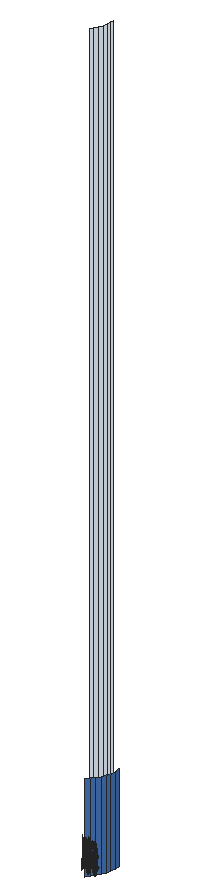
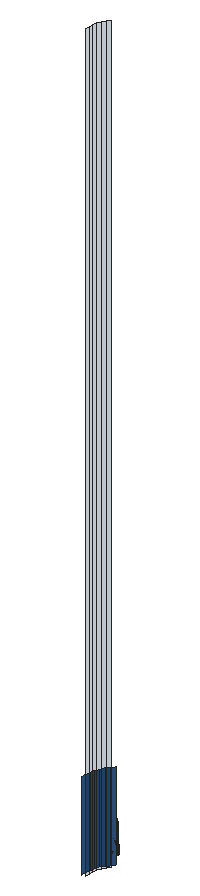
# SketchUp Ruby script. Lengths in inches.
U = 1.inch
M = Sketchup.active_model
def pt(a) = Geom::Point3d.new(a.map { |v| v * U })
def face(e, loops, mat)
  f = e.add_face(loops[0].map { |a| pt(a) })
  loops[1..].each { |l| e.add_face(l.map { |a| pt(a) }).erase! }
  f.material = f.back_material = mat if mat
  f
end
# faces: each face lists its corners as indices into pts; further lists are holes
def faces(e, pts, list, mat = nil) = list.each { |f| face(e, (f[0].is_a?(Array) ? f : [f]).map { |l| l.map { |i| pts[i] } }, mat) }
# xy, xz, yz: faces in a plane at the given z, y or x. An outline is a flat list of corners, or four numbers for a rectangle; further outlines are holes
def ring(l) = l.size == 4 ? [[l[0], l[1]], [l[2], l[1]], [l[2], l[3]], [l[0], l[3]]] : l.each_slice(2).to_a
def flat(e, list, mat, &to3) = list.each { |f| face(e, (f[0].is_a?(Array) ? f : [f]).map { |l| ring(l).map { |u, v| to3.(u, v) } }, mat) }
def xy(e, z, list, mat = nil) = flat(e, list, mat) { |x, y| [x, y, z] }
def xz(e, y, list, mat = nil) = flat(e, list, mat) { |x, z| [x, y, z] }
def yz(e, x, list, mat = nil) = flat(e, list, mat) { |y, z| [x, y, z] }
def lines(e, pts, list) = list.each { |a, b| e.add_line(pt(pts[a]), pt(pts[b])) }
# prism: a flat outline (further loops are holes) pulled along v
def prism(e, loops, v, mat = nil)
  f = face(e, loops, mat); d = Geom::Vector3d.new(v.map { |x| x * U })
  f.pushpull(f.normal.samedirection?(d) ? d.length : -d.length)
end
def box(e, o, s, mat = nil) = prism(e, [[o, [o[0] + s[0], o[1], o[2]], [o[0] + s[0], o[1] + s[1], o[2]], [o[0], o[1] + s[1], o[2]]]], [0, 0, s[2]], mat)
def at(x, y, z, deg = 0) = Geom::Transformation.translation(pt([x, y, z])) * Geom::Transformation.rotation(ORIGIN, Z_AXIS, deg.degrees)
def axes(o, x, y, z) = Geom::Transformation.new([*x, 0, *y, 0, *z, 0, *pt(o).to_a, 1])
def part(name) = M.definitions.add(name)
# library, detail: a bought-in or finely detailed component or shape, given as its bounding box
def library(name, o, s) = part(name).tap { |d| box(d.entities, o, s) }
def detail(e, o, s) = box(e.add_group.entities, o, s)
def put(e, d, t, mat = nil) = e.add_instance(d, t).tap { |i| i.material = mat if mat }
def group(e, t, mat = nil) = e.add_group.tap { |g| g.transformation = t; g.material = mat if mat }.entities
root = M.entities
M.materials.add("Glass_Basic_1").color = [0, 47, 91]
M.materials["Glass_Basic_1"].alpha = 0.25
M.materials.add("Glass_Mirror_01").color = [71, 118, 185]
M.materials.add("LightPink_Translucent").color = [144, 107, 117]
M.materials["LightPink_Translucent"].alpha = 0.75
c1 = part("blade")
p = [[2.15,0.21,22],[0,0.17,0],[0.09,0.45,0],[2.18,0.31,22],[2.29,0.31,22],[0.38,0.45,0],
  [2.48,0.24,33],[2.49,0.24,33],[2.48,0.22,33]]
faces(c1.entities,p,[[0,1,2,3],[4,5,2,3],[6,3,4,7],[8,0,3,6]])
c2 = part("seeds")
p = [[0.3,-0.1,1.38],[-0.01,-0.03,1.59],[-0.01,-0.03,0.03],[0.14,-0.07,-0.07],[0.29,-0.03,3],[0.15,0.01,3.11]]
faces(c2.entities,p,[[0,1,2,3],[1,0,4,5]],"LightPink_Translucent")
c3 = part("blade with seeds")
put(c3.entities,c1,at(0,0,0))
put(c3.entities,c2,axes([2.4,0.25,30.99],[1.5799,-0.05474,1.17369],[-0.12525,1.92788,0.29478],[-0.07173,-0.02425,1.56792]))
yz(root,371.64,[[77.78,-24,85.69,1482]],"Glass_Basic_1")
yz(root,380.64,[[77.22,-24,86.26,150]],"Glass_Mirror_01")
p = [[364.26,35.84,-24],[364.26,35.84,150],[358.07,29.25,150],[358.07,29.25,-24],[369.57,43.16,-24],[369.57,43.16,150],
  [357.31,41.59,1482],[361.96,47.99,1482],[361.96,47.99,-24],[357.31,41.59,-24],[373.93,51.08,-24],[373.93,51.08,150],
  [365.77,54.92,1482],[365.77,54.92,-24],[377.26,59.49,-24],[377.26,59.49,150],[368.68,62.28,1482],[368.68,62.28,-24],
  [379.51,68.25,-24],[379.51,68.25,150],[370.65,69.9375,1482],[370.65,69.9375,-24],[380.64,77.22,-24],[380.64,77.22,150],
  [371.64,77.78,1482],[371.64,77.78,-24]]
faces(root,p,[[0,1,2,3],[4,5,1,0],[10,11,5,4],[14,15,11,10],[18,19,15,14],[22,23,19,18]],"Glass_Mirror_01")
faces(root,p,[[6,7,8,9],[7,12,13,8],[12,16,17,13],[16,20,21,17],[20,24,25,21]],"Glass_Basic_1")
put(root,c3,axes([370.71,21.25,-11.3125],[0.08291,0.40636,-0.30978],[-0.32928,0.11539,0.30978],[0.06638,0.04686,1.38974]))
put(root,c3,axes([358.8,22.875,-5.59],[0.12963,0.31798,0.0643],[-0.23638,0.15564,0.50621],[0.1042,-0.03071,0.77189]))
put(root,c3,axes([371.28,22.875,-8.61],[0.12963,0.31798,0.0643],[-0.23638,0.15564,0.50621],[0.1042,-0.03071,0.77189]))
put(root,c3,axes([370.05,22.16,-10.96],[-0.44609,-0.09826,0.49198],[0.09078,-0.55493,0.19306],[0.06519,0.05359,1.70813]))
put(root,c3,axes([358.78,22.76,-5.59],[-0.09971,0.42522,0.48003],[-0.32782,-0.1454,0.3958],[0.12892,-0.02555,0.9933]))
put(root,c3,axes([371.25,22.76,-8.61],[-0.09971,0.42522,0.48003],[-0.32782,-0.1454,0.3958],[0.12892,-0.02555,0.9933]))
put(root,c3,axes([369.69,23.53,-11.14],[-0.11516,-0.40207,0],[0.32884,-0.1408,0],[0,0,1.54371]))
put(root,c3,axes([383.12,23.53,-11.01],[-0.11516,-0.40207,0],[0.32884,-0.1408,0],[0,0,1.54371]))
put(root,c3,axes([369.47,23.15,-10.73],[-0.06809,0.4162,0.1448],[-0.33266,-0.07225,-0.41347],[-0.06054,-0.04274,1.26744]))
put(root,c3,axes([382.9,23.15,-10.59],[-0.06809,0.4162,0.1448],[-0.33266,-0.07225,-0.41347],[-0.06054,-0.04274,1.26744]))
put(root,c3,axes([368.18,22.07,-8.29],[0.29332,0.1301,0.35414],[-0.08555,0.37955,-0.4572],[-0.11809,0.0348,0.87481]))
put(root,c3,axes([381.61,22.07,-8.16],[0.29332,0.1301,0.35414],[-0.08555,0.37955,-0.4572],[-0.11809,0.0348,0.87481]))
put(root,c3,axes([357.65,23.48,-8.14],[0.37054,-0.15823,-0.19198],[0.1302,0.45581,0.00008],[0.0409,-0.01749,1.73897]))
put(root,c3,axes([370.125,23.48,-11.16],[0.37054,-0.15823,-0.19198],[0.1302,0.45581,0.00008],[0.0409,-0.01749,1.73897]))
put(root,c3,axes([370.25,23.67,-10.87],[0.10196,-0.46348,0.17642],[0.3731,0.13116,0.35086],[-0.06445,0.00226,1.60407]))
put(root,c3,axes([383.68,23.67,-10.74],[0.10196,-0.46348,0.17642],[0.3731,0.13116,0.35086],[-0.06445,0.00226,1.60407]))
put(root,c3,axes([370.17,22.62,-11.13],[0.24637,0.30123,0],[-0.24637,0.30123,0],[0,0,1.69266]))
put(root,c3,axes([368.77,22.05,-10],[0.10032,-0.06746,1.77064],[0.0346,0.47103,0.13857],[-0.2173,0.0625,0.63284]))
put(root,c3,axes([382.19,22.05,-9.87],[0.10032,-0.06746,1.77064],[0.0346,0.47103,0.13857],[-0.2173,0.0625,0.63284]))
put(root,c3,axes([370.83,22.48,-10.87],[-0.2773,-0.3397,0.17642],[0.27945,-0.32949,0.35086],[-0.03063,0.06937,1.60407]))
put(root,c3,axes([384.26,22.48,-10.74],[-0.2773,-0.3397,0.17642],[0.27945,-0.32949,0.35086],[-0.03063,0.06937,1.60407]))
put(root,c3,axes([357.85,21.97,-8.26],[0.36714,0.07646,-0.62353],[-0.07747,0.47163,-0.16365],[0.10956,0.05715,1.37633]))
put(root,c3,axes([370.32,21.97,-11.28],[0.36714,0.07646,-0.62353],[-0.07747,0.47163,-0.16365],[0.10956,0.05715,1.37633]))
put(root,c3,axes([359.47,22.79,-7.56],[-0.21807,0.07699,1.1486],[0.10265,-0.31819,0.84392],[0.11568,0.02177,0.25299]))
put(root,c3,axes([371.94,22.79,-10.58],[-0.21807,0.07699,1.1486],[0.10265,-0.31819,0.84392],[0.11568,0.02177,0.25299]))
put(root,c3,axes([369.61,23.71,-11.15],[-0.35581,-0.20937,0],[0.17124,-0.43505,0],[0,0,1.62707]))
put(root,c3,axes([383.04,23.71,-11.02],[-0.35581,-0.20937,0],[0.17124,-0.43505,0],[0,0,1.62707]))
put(root,c3,axes([369.91,23.16,-10.88],[-0.34464,-0.37536,-0.25192],[0.29,-0.42149,0.5513],[-0.0928,0.04391,1.68216]))
put(root,c3,axes([383.33,23.16,-10.75],[-0.34464,-0.37536,-0.25192],[0.29,-0.42149,0.5513],[-0.0928,0.04391,1.68216]))
put(root,c3,axes([369,23.875,-10.86],[0.33032,0.23318,0.49651],[-0.19744,0.41812,0],[-0.07523,-0.05311,1.57504]))
put(root,c3,axes([382.43,23.875,-10.73],[0.33032,0.23318,0.49651],[-0.19744,0.41812,0],[-0.07523,-0.05311,1.57504]))
put(root,c3,axes([370.16,22.26,-10.625],[0.17124,-0.42022,0.44739],[0.35581,0.20224,-0.21531],[0,0.09687,1.43643]))
put(root,c3,axes([359.37,24.14,-5.61],[-0.03191,-0.04083,1.77383],[0.06981,-0.43764,-0.16761],[0.12571,-0.02796,0.31391]))
put(root,c3,axes([371.84,24.14,-8.63],[-0.03191,-0.04083,1.77383],[0.06981,-0.43764,-0.16761],[0.12571,-0.02796,0.31391]))
put(root,c3,axes([367.6875,22.37,-8.625],[-0.05763,0.06055,1.74944],[0.0049,0.44239,-0.27667],[-0.13211,0.05753,0.14031]))
put(root,c3,axes([381.11,22.37,-8.5],[-0.05763,0.06055,1.74944],[0.0049,0.44239,-0.27667],[-0.13211,0.05753,0.14031]))
put(root,c3,axes([370.1,22.5,-11.05],[0,0.53934,-0.05637],[-0.44133,0,0],[0,0.01695,1.79368]))
put(root,c3,axes([368.07,22.31,-8.66],[-0.09562,0.42421,-0.51099],[-0.32782,-0.1454,-0.3958],[-0.13199,0.0389,0.97773]))
put(root,c3,axes([381.5,22.31,-8.53],[-0.09562,0.42421,-0.51099],[-0.32782,-0.1454,-0.3958],[-0.13199,0.0389,0.97773]))
put(root,c3,axes([368.06,21.94,-8.31],[0.17758,0.42229,-0.1216],[-0.31518,0.20752,-0.67495],[-0.13282,0.05572,1.02557]))
put(root,c3,axes([381.48,21.94,-8.18],[0.17758,0.42229,-0.1216],[-0.31518,0.20752,-0.67495],[-0.13282,0.05572,1.02557]))
put(root,c3,axes([357.66,22.12,-8.11],[0.21202,0.39143,-0.44739],[-0.32115,0.27564,0.21531],[0.06861,0.04843,1.43643]))
put(root,c3,axes([370.13,22.12,-11.13],[0.21202,0.39143,-0.44739],[-0.32115,0.27564,0.21531],[0.06861,0.04843,1.43643]))
put(root,c3,axes([359.09,23.78,-6.39],[-0.06755,-0.39203,-0.03492],[0.31928,-0.09013,-0.15832],[0.06667,0.02485,0.52218]))
put(root,c3,axes([371.56,23.78,-9.41],[-0.06755,-0.39203,-0.03492],[0.31928,-0.09013,-0.15832],[0.06667,0.02485,0.52218]))
put(root,c3,axes([368.81,24.12,-10.97],[-0.22066,0.46731,0],[-0.36918,-0.26061,-0.51607],[-0.08408,-0.05936,1.63711]))
put(root,c3,axes([382.23,24.12,-10.84],[-0.22066,0.46731,0],[-0.36918,-0.26061,-0.51607],[-0.08408,-0.05936,1.63711]))
put(root,c3,axes([358.26,23.76,-5.29],[0.0189,-0.47427,-0.1216],[0.35781,0.01296,-0.67495],[0.13781,0.03295,1.02557]))
put(root,c3,axes([370.74,23.76,-8.31],[0.0189,-0.47427,-0.1216],[0.35781,0.01296,-0.67495],[0.13781,0.03295,1.02557]))
put(root,c3,axes([371.0625,22.5,-10.86],[0,-0.46636,0.49651],[0.39487,0,0],[0,0.10622,1.57504]))
put(root,c3,axes([370.07,22.85,-10.625],[0.38326,-0.02879,0.44739],[0.03466,0.47788,-0.21531],[-0.06861,0.04843,1.43643]))
put(root,c3,axes([383.5,22.85,-10.49],[0.38326,-0.02879,0.44739],[0.03466,0.47788,-0.21531],[-0.06861,0.04843,1.43643]))
put(root,c3,axes([370.3125,22.36,-10.73],[0.32884,-0.136,0.1448],[0.11516,0.38837,-0.41347],[0,0.08547,1.26744]))
put(root,c3,axes([358.21,23.58,-5.27],[-0.20082,-0.29199,0.35414],[0.2293,-0.2764,-0.4572],[0.1165,0.04206,0.87481]))
put(root,c3,axes([370.68,23.58,-8.29],[-0.20082,-0.29199,0.35414],[0.2293,-0.2764,-0.4572],[0.1165,0.04206,0.87481]))
put(root,c3,axes([369.73,23.08,-11.13],[-0.38326,0.02879,-0.44739],[-0.03466,-0.47788,0.21531],[-0.06861,0.04843,1.43643]))
put(root,c3,axes([383.16,23.08,-11],[-0.38326,0.02879,-0.44739],[-0.03466,-0.47788,0.21531],[-0.06861,0.04843,1.43643]))
put(root,c3,axes([359.06,23.3,-7.73],[-0.085,-0.1147,1.43002],[0.1106,-0.37943,-0.30754],[0.17198,0.0514,0.61141]))
put(root,c3,axes([371.53,23.3,-10.75],[-0.085,-0.1147,1.43002],[0.1106,-0.37943,-0.30754],[0.17198,0.0514,0.61141]))
put(root,c3,axes([370.02,23.72,-11.14],[0.35581,0.20937,0],[-0.17124,0.43505,0],[0,0,1.74954]))
put(root,c3,axes([358.57,23.48,-5.61],[0.07571,-0.00789,1.74944],[0.20767,-0.36231,-0.27667],[0.13467,0.04783,0.14031]))
put(root,c3,axes([371.05,23.48,-8.625],[0.07571,-0.00789,1.74944],[0.20767,-0.36231,-0.27667],[0.13467,0.04783,0.14031]))
put(root,c3,axes([370.16,24.19,-11.15],[-0.21791,-0.46895,-0.05142],[0.36918,-0.26061,0.51607],[-0.09097,0.04465,1.6363]))
put(root,c3,axes([383.58,24.19,-11.02],[-0.21791,-0.46895,-0.05142],[0.36918,-0.26061,0.51607],[-0.09097,0.04465,1.6363]))
put(root,c3,axes([370.08,23.05,-10.73],[0.26075,0.2802,0.1448],[-0.2175,0.31612,-0.41347],[-0.06054,0.04274,1.26744]))
put(root,c3,axes([383.51,23.05,-10.59],[0.26075,0.2802,0.1448],[-0.2175,0.31612,-0.41347],[-0.06054,0.04274,1.26744]))
put(root,c3,axes([368.02,23.125,-8.61],[-0.08753,-0.42921,0.48003],[0.34336,-0.07449,0.3958],[-0.1012,0.10094,0.9933]))
put(root,c3,axes([381.45,23.125,-8.48],[-0.08753,-0.42921,0.48003],[0.34336,-0.07449,0.3958],[-0.1012,0.10094,0.9933]))
put(root,c3,axes([367.95,23.04,-8.61],[-0.2423,-0.19613,0.0643],[0.14107,-0.2793,0.50621],[-0.07768,0.0903,0.77189]))
put(root,c3,axes([381.38,23.04,-8.48],[-0.2423,-0.19613,0.0643],[0.14107,-0.2793,0.50621],[-0.07768,0.0903,0.77189]))
put(root,c3,axes([368.0625,22.52,-9.47],[0.12246,-0.09864,1.71376],[0.1031,0.45582,0.13857],[-0.19225,0.10302,0.73262]))
put(root,c3,axes([381.49,22.52,-9.33],[0.12246,-0.09864,1.71376],[0.1031,0.45582,0.13857],[-0.19225,0.10302,0.73262]))
put(root,c3,axes([358.28,23.54,-5.34],[0.35281,0.01123,-0.71045],[-0.0237,0.47284,0.08574],[0.14947,0.0499,1.00501]))
put(root,c3,axes([370.75,23.54,-8.36],[0.35281,0.01123,-0.71045],[-0.0237,0.47284,0.08574],[0.14947,0.0499,1.00501]))
put(root,c3,axes([370.36,23.91,-10.86],[0.33032,-0.23318,0.49651],[0.19744,0.41812,0],[-0.07523,0.05311,1.57504]))
put(root,c3,axes([383.78,23.91,-10.73],[0.33032,-0.23318,0.49651],[0.19744,0.41812,0],[-0.07523,0.05311,1.57504]))
put(root,c3,axes([369.89,23.55,-11.05],[0.15345,0.53576,-0.06012],[-0.43845,0.18773,0],[0.00536,0.01871,1.72173]))
put(root,c3,axes([370.06,24.125,-11.3125],[-0.32928,-0.11539,-0.30978],[0.08291,-0.40636,0.30978],[-0.06638,0.04686,1.38974]))
put(root,c3,axes([383.48,24.125,-11.18],[-0.32928,-0.11539,-0.30978],[0.08291,-0.40636,0.30978],[-0.06638,0.04686,1.38974]))
put(root,c3,axes([367.68,23.3,-10.75],[0.12266,0.03828,1.43002],[0.07906,0.39104,-0.30754],[-0.16661,0.0732,0.61141]))
put(root,c3,axes([381.11,23.3,-10.62],[0.12266,0.03828,1.43002],[0.07906,0.39104,-0.30754],[-0.16661,0.0732,0.61141]))
put(root,c3,axes([368.23,22.98,-8.29],[0.30722,-0.06665,0.35414],[0.08112,0.381,-0.4572],[-0.08804,0.10234,0.87481]))
put(root,c3,axes([381.66,22.98,-8.16],[0.30722,-0.06665,0.35414],[0.08112,0.381,-0.4572],[-0.08804,0.10234,0.87481]))
put(root,c3,axes([358.86,22.58,-7.95],[0.44133,0,0],[0,0.52122,-0.51607],[0,0.11871,1.63711]))
put(root,c3,axes([371.33,22.58,-10.97],[0.44133,0,0],[0,0.52122,-0.51607],[0,0.11871,1.63711]))
put(root,c3,axes([367.05,22.8125,-8.63],[0.04504,0.01251,1.77383],[0.13934,0.41205,-0.16761],[-0.0922,0.10815,0.31391]))
put(root,c3,axes([380.47,22.8125,-8.5],[0.04504,0.01251,1.77383],[0.13934,0.41205,-0.16761],[-0.0922,0.10815,0.31391]))
put(root,c3,axes([371.15,22.84,-11.14],[-0.44111,-0.00373,-0.04976],[0,-0.52122,0.49943],[-0.01386,0.11865,1.58352]))
put(root,c3,axes([370.2,22.39,-10.68],[0.39748,0.22252,-0.29095],[-0.19139,0.46966,-0.50002],[0.01249,0.11531,1.59708]))
put(root,c3,axes([367.43,24.12,-10.58],[0.14709,-0.21136,1.1486],[0.05804,0.3346,0.84392],[-0.1063,0.05991,0.25299]))
put(root,c3,axes([380.85,24.12,-10.45],[0.14709,-0.21136,1.1486],[0.05804,0.3346,0.84392],[-0.1063,0.05991,0.25299]))
put(root,c3,axes([358.49,23.73,-5.8],[0.20082,0.29199,-0.35414],[-0.2293,0.2764,0.4572],[0.1165,0.04206,0.87481]))
put(root,c3,axes([370.97,23.73,-8.82],[0.20082,0.29199,-0.35414],[-0.2293,0.2764,0.4572],[0.1165,0.04206,0.87481]))
put(root,c3,axes([371.0625,22.92,-11.3125],[-0.24637,0.29097,-0.30978],[-0.24637,-0.29097,0.30978],[0,0.09372,1.38974]))
put(root,c3,axes([370,22.95,-10.68],[0.04113,0.53214,-0.29095],[-0.42835,0.03218,-0.50002],[-0.07543,0.07088,1.59708]))
put(root,c3,axes([383.43,22.95,-10.55],[0.04113,0.53214,-0.29095],[-0.42835,0.03218,-0.50002],[-0.07543,0.07088,1.59708]))
put(root,c3,axes([358.39,23.84,-5.59],[-0.01777,0.35463,0.0643],[-0.26836,-0.00972,0.50621],[0.1028,0.03711,0.77189]))
put(root,c3,axes([370.86,23.84,-8.61],[-0.01777,0.35463,0.0643],[-0.26836,-0.00972,0.50621],[0.1028,0.03711,0.77189]))
put(root,c3,axes([370.16,22.74,-11.13],[-0.17124,0.42022,-0.44739],[-0.35581,-0.20224,0.21531],[0,0.09687,1.43643]))
put(root,c3,axes([383.58,22.74,-11],[-0.17124,0.42022,-0.44739],[-0.35581,-0.20224,0.21531],[0,0.09687,1.43643]))
put(root,c3,axes([367.98,23.21,-8.82],[-0.30722,0.06665,-0.35414],[-0.08112,-0.381,0.4572],[-0.08804,0.10234,0.87481]))
put(root,c3,axes([381.41,23.21,-8.68],[-0.30722,0.06665,-0.35414],[-0.08112,-0.381,0.4572],[-0.08804,0.10234,0.87481]))
put(root,c3,axes([358.41,23.73,-5.59],[-0.26024,0.30729,0.48003],[-0.22444,-0.32634,0.3958],[0.1221,0.05668,0.9933]))
put(root,c3,axes([370.89,23.73,-8.61],[-0.26024,0.30729,0.48003],[-0.22444,-0.32634,0.3958],[0.1221,0.05668,0.9933]))
put(root,c3,axes([367.53,24.0625,-7.7],[0.31145,0.12449,-0.06488],[-0.0958,0.38314,-0.29416],[-0.05094,0.05817,0.97024]))
put(root,c3,axes([380.96,24.0625,-7.56],[0.31145,0.12449,-0.06488],[-0.0958,0.38314,-0.29416],[-0.05094,0.05817,0.97024]))
put(root,c3,axes([369.74,23.35,-11.28],[-0.23773,0.35053,-0.62353],[-0.29532,-0.31785,-0.16365],[-0.09526,0.08744,1.37633]))
put(root,c3,axes([383.17,23.35,-11.15],[-0.23773,0.35053,-0.62353],[-0.29532,-0.31785,-0.16365],[-0.09526,0.08744,1.37633]))
put(root,c3,axes([357.59,24.09,-5.27],[-0.05451,-0.37564,0.35414],[0.31161,-0.09919,-0.4572],[0.0837,0.10765,0.87481]))
put(root,c3,axes([370.0625,24.09,-8.29],[-0.05451,-0.37564,0.35414],[0.31161,-0.09919,-0.4572],[0.0837,0.10765,0.87481]))
put(root,c3,axes([370.17,23.94,-11.01],[0.44186,0.15158,0.30756],[-0.11054,0.54181,-0.36492],[-0.07313,0.06781,1.64885]))
put(root,c3,axes([383.59,23.94,-10.88],[0.44186,0.15158,0.30756],[-0.11054,0.54181,-0.36492],[-0.07313,0.06781,1.64885]))
put(root,c3,axes([370.14,24.31,-11.32],[-0.33032,0.23318,-0.49651],[-0.19744,-0.41812,0],[-0.07523,0.05311,1.57504]))
put(root,c3,axes([383.56,24.31,-11.19],[-0.33032,0.23318,-0.49651],[-0.19744,-0.41812,0],[-0.07523,0.05311,1.57504]))
put(root,c3,axes([371.23,22.93,-11.32],[0,0.46636,-0.49651],[-0.39487,0,0],[0,0.10622,1.57504]))
put(root,c3,axes([357.77,22.98,-6.45],[-0.1311,-0.08035,1.71376],[0.27131,-0.33708,0.13857],[0.16909,0.15206,0.73262]))
put(root,c3,axes([370.25,22.98,-9.47],[-0.1311,-0.08035,1.71376],[0.27131,-0.33708,0.13857],[0.16909,0.15206,0.73262]))
put(root,c3,axes([357.8,21.92,-5.85],[-0.30498,-0.24231,1.38283],[0.32203,-0.37727,0.59665],[0.0984,0.22736,1.33663]))
put(root,c3,axes([370.27,21.92,-8.87],[-0.30498,-0.24231,1.38283],[0.32203,-0.37727,0.59665],[0.0984,0.22736,1.33663]))
put(root,c3,axes([368.07,22.95,-8.31],[0.32648,0.25715,-0.1216],[-0.18809,0.3724,-0.67495],[-0.09224,0.12945,1.02557]))
put(root,c3,axes([381.5,22.95,-8.18],[0.32648,0.25715,-0.1216],[-0.18809,0.3724,-0.67495],[-0.09224,0.12945,1.02557]))
put(root,c3,axes([358.26,23.9,-7.56],[-0.19872,-0.13409,1.1486],[0.2566,-0.13625,0.84392],[0.06921,0.11541,0.25299]))
put(root,c3,axes([370.73,23.9,-10.58],[-0.19872,-0.13409,1.1486],[0.2566,-0.13625,0.84392],[0.06921,0.11541,0.25299]))
put(root,c3,axes([357.56,24.28,-5.29],[0.21031,-0.39918,-0.1216],[0.30457,0.22997,-0.67495],[0.10587,0.11278,1.02557]))
put(root,c3,axes([370.03,24.28,-8.31],[0.21031,-0.39918,-0.1216],[0.30457,0.22997,-0.67495],[0.10587,0.11278,1.02557]))
put(root,c3,axes([368.51,22.83,-9.47],[0.08815,-0.14329,1.71376],[0.22258,0.38678,0.13857],[-0.15267,0.17614,0.73262]))
put(root,c3,axes([381.9375,22.83,-9.33],[0.08815,-0.14329,1.71376],[0.22258,0.38678,0.13857],[-0.15267,0.17614,0.73262]))
put(root,c3,axes([368.23,23.25,-8.66],[0.09067,0.42583,-0.51099],[-0.34336,0.07449,-0.3958],[-0.0984,0.11438,0.97773]))
put(root,c3,axes([381.66,23.25,-8.53],[0.09067,0.42583,-0.51099],[-0.34336,0.07449,-0.3958],[-0.0984,0.11438,0.97773]))
put(root,c3,axes([368.65,23.74,-8.29],[0.23881,-0.24554,0.35414],[0.22606,0.28036,-0.4572],[-0.0344,0.14245,0.87481]))
put(root,c3,axes([382.07,23.74,-8.16],[0.23881,-0.24554,0.35414],[0.22606,0.28036,-0.4572],[-0.0344,0.14245,0.87481]))
put(root,c3,axes([370.43,24.24,-10.97],[0.22066,0.46731,0],[-0.36918,0.26061,-0.51607],[-0.08408,0.05936,1.63711]))
put(root,c3,axes([383.86,24.24,-10.84],[0.22066,0.46731,0],[-0.36918,0.26061,-0.51607],[-0.08408,0.05936,1.63711]))
put(root,c3,axes([357.28,24.61,-5.61],[0.00104,-0.05646,1.77383],[0.30246,-0.2491,-0.16761],[0.10506,0.08891,0.31391]))
put(root,c3,axes([369.76,24.61,-8.63],[0.00104,-0.05646,1.77383],[0.30246,-0.2491,-0.16761],[0.10506,0.08891,0.31391]))
put(root,c3,axes([358.3125,24.4,-8.83],[0.02571,-0.06733,1.76342],[0.32373,-0.19829,-0.26939],[0.09815,0.10263,0.30037]))
put(root,c3,axes([370.79,24.4,-11.85],[0.02571,-0.06733,1.76342],[0.32373,-0.19829,-0.26939],[0.09815,0.10263,0.30037]))
put(root,c3,axes([370.25,22.39,-10.5],[-0.00964,-0.43909,1.41272],[0.43635,0.11382,0.59816],[-0.1032,0.24027,1.3335]))
put(root,c3,axes([383.67,22.39,-10.37],[-0.00964,-0.43909,1.41272],[0.43635,0.11382,0.59816],[-0.1032,0.24027,1.3335]))
put(root,c3,axes([370.36,22.87,-11.25],[0.12941,0.42699,-0.69212],[-0.37279,0.15378,-0.18165],[0.0143,0.14459,1.52773]))
put(root,c3,axes([368.43,23.96,-8.61],[-0.29004,-0.02173,0.0643],[0.00795,-0.32812,0.50621],[-0.03035,0.12569,0.77189]))
put(root,c3,axes([381.85,23.96,-8.48],[-0.29004,-0.02173,0.0643],[0.00795,-0.32812,0.50621],[-0.03035,0.12569,0.77189]))
put(root,c3,axes([367.8125,24.34,-11.85],[0.04734,0.04659,1.76342],[0.08027,0.4317,-0.26939],[-0.10492,0.09206,0.30037]))
put(root,c3,axes([381.24,24.34,-11.72],[0.04734,0.04659,1.76342],[0.08027,0.4317,-0.26939],[-0.10492,0.09206,0.30037]))
put(root,c3,axes([368.52,23.99,-8.61],[-0.25132,-0.3182,0.48003],[0.2669,-0.27442,0.3958],[-0.04636,0.14929,0.9933]))
put(root,c3,axes([381.95,23.99,-8.48],[-0.25132,-0.3182,0.48003],[0.2669,-0.27442,0.3958],[-0.04636,0.14929,0.9933]))
put(root,c3,axes([357.81,24.08,-5.64],[0.34827,-0.11086,-0.51099],[0.06092,0.41983,-0.3958],[0.09354,0.12031,0.97773]))
put(root,c3,axes([370.28,24.08,-8.66],[0.34827,-0.11086,-0.51099],[0.06092,0.41983,-0.3958],[0.09354,0.12031,0.97773]))
put(root,c3,axes([369.32,24.14,-8.29],[0.1064,-0.35863,0.35414],[0.31043,0.1046,-0.4572],[0.02846,0.14439,0.87481]))
put(root,c3,axes([358.29,24.51,-7.65],[-0.22633,-0.01463,1.0506],[0.14947,-0.31064,0.58006],[0.08941,0.11036,0.8241]))
put(root,c3,axes([370.76,24.51,-10.67],[-0.22633,-0.01463,1.0506],[0.14947,-0.31064,0.58006],[0.08941,0.11036,0.8241]))
put(root,c3,axes([357.64,24.43,-5.59],[-0.16041,0.29625,0.0643],[-0.22843,-0.17248,0.50621],[0.07385,0.09498,0.77189]))
put(root,c3,axes([370.11,24.43,-8.61],[-0.16041,0.29625,0.0643],[-0.22843,-0.17248,0.50621],[0.07385,0.09498,0.77189]))
put(root,c3,axes([369.73,25.42,-7.7],[0.2439,-0.26754,-0.06488],[0.22348,0.29302,-0.29416],[0.01573,0.08303,0.97024]))
put(root,c3,axes([357.7,24.34,-5.59],[-0.35104,0.10702,0.48003],[-0.06092,-0.41983,0.3958],[0.08256,0.12373,0.9933]))
put(root,c3,axes([370.18,24.34,-8.61],[-0.35104,0.10702,0.48003],[-0.06092,-0.41983,0.3958],[0.08256,0.12373,0.9933]))
put(root,c3,axes([368.45,23.19,-9.47],[0.06572,-0.16029,1.71376],[0.27569,0.33172,0.13857],[-0.12437,0.20675,0.73262]))
put(root,c3,axes([381.87,23.19,-9.33],[0.06572,-0.16029,1.71376],[0.27569,0.33172,0.13857],[-0.12437,0.20675,0.73262]))
put(root,c3,axes([357.55,23.75,-7.73],[0.00623,-0.15459,1.43002],[0.29764,-0.17268,-0.30754],[0.09188,0.18503,0.61141]))
put(root,c3,axes([370.02,23.75,-10.75],[0.00623,-0.15459,1.43002],[0.29764,-0.17268,-0.30754],[0.09188,0.18503,0.61141]))
put(root,c3,axes([369.22,24.47,-8.61],[-0.26007,0.1585,0.0643],[-0.12729,-0.28902,0.50621],[0.02512,0.1274,0.77189]))
put(root,c3,axes([382.64,24.47,-8.48],[-0.26007,0.1585,0.0643],[-0.12729,-0.28902,0.50621],[0.02512,0.1274,0.77189]))
put(root,c3,axes([368.52,24.09,-8.82],[-0.23881,0.24554,-0.35414],[-0.22606,-0.28036,0.4572],[-0.0344,0.14245,0.87481]))
put(root,c3,axes([381.95,24.09,-8.68],[-0.23881,0.24554,-0.35414],[-0.22606,-0.28036,0.4572],[-0.0344,0.14245,0.87481]))
put(root,c3,axes([367.7,24.02,-8.625],[-0.00877,0.09229,1.74944],[0.24897,0.32105,-0.27667],[-0.06518,0.15182,0.14031]))
put(root,c3,axes([381.125,24.02,-8.5],[-0.00877,0.09229,1.74944],[0.24897,0.32105,-0.27667],[-0.06518,0.15182,0.14031]))
put(root,c3,axes([368.49,23.81,-7.94],[0.3879,0.02311,-0.13498],[-0.0106,0.43749,-0.74919],[-0.02694,0.1685,1.13838]))
put(root,c3,axes([381.92,23.81,-7.8125],[0.3879,0.02311,-0.13498],[-0.0106,0.43749,-0.74919],[-0.02694,0.1685,1.13838]))
put(root,c3,axes([369.21,24.3,-8.31],[0.34538,-0.21713,-0.1216],[0.16972,0.38536,-0.67495],[0.04557,0.16239,1.02557]))
put(root,c3,axes([369.3125,24.4375,-8.28],[-0.34777,-0.12192,0.53283],[0.11892,-0.40083,0.43934],[0.0209,0.15763,1.10256]))
put(root,c3,axes([382.74,24.4375,-8.15],[-0.34777,-0.12192,0.53283],[0.11892,-0.40083,0.43934],[0.0209,0.15763,1.10256]))
put(root,c3,axes([368.67,25.04,-10.58],[-0.00913,-0.2773,1.1486],[0.22824,0.19778,0.84392],[-0.04489,0.13217,0.25299]))
put(root,c3,axes([382.1,25.04,-10.45],[-0.00913,-0.2773,1.1486],[0.22824,0.19778,0.84392],[-0.04489,0.13217,0.25299]))
put(root,c3,axes([369.27,24.38,-11.85],[0.05712,-0.02538,1.76342],[0.34359,0.13968,-0.26939],[0.01005,0.15742,0.30037]))
put(root,c3,axes([382.7,24.38,-11.72],[0.05712,-0.02538,1.76342],[0.34359,0.13968,-0.26939],[0.01005,0.15742,0.30037]))
put(root,c3,axes([368.76,23.97,-8.34],[0.25266,0.31335,-0.5672],[-0.2669,0.27442,-0.43934],[-0.03844,0.15921,1.08528]))
put(root,c3,axes([382.18,23.97,-8.21],[0.25266,0.31335,-0.5672],[-0.2669,0.27442,-0.43934],[-0.03844,0.15921,1.08528]))
put(root,c3,axes([368.48,24.44,-10.52],[0.32063,-0.08258,0.06507],[0.07371,0.33271,-0.86304],[-0.02033,0.16842,0.7736]))
put(root,c3,axes([381.91,24.44,-10.39],[0.32063,-0.08258,0.06507],[0.07371,0.33271,-0.86304],[-0.02033,0.16842,0.7736]))
put(root,c3,axes([369.51,24.28,-8.66],[0.34695,0.11691,-0.51099],[-0.11892,0.40083,-0.3958],[0.03181,0.16138,0.97773]))
put(root,c3,axes([357.23,23.45,-6.45],[-0.08068,-0.14973,1.71376],[0.3728,-0.12606,0.13857],[0.08426,0.23506,0.73262]))
put(root,c3,axes([369.71,23.45,-9.47],[-0.08068,-0.14973,1.71376],[0.3728,-0.12606,0.13857],[0.08426,0.23506,0.73262]))
put(root,c3,axes([369.35,24.52,-8.82],[-0.1064,0.35863,-0.35414],[-0.31043,-0.1046,0.4572],[0.02846,0.14439,0.87481]))
put(root,c3,axes([382.78,24.52,-8.68],[-0.1064,0.35863,-0.35414],[-0.31043,-0.1046,0.4572],[0.02846,0.14439,0.87481]))
put(root,c3,axes([368.68,23.83,-8],[-0.00918,0.43138,-0.7886],[-0.38672,-0.02897,0.09517],[-0.04081,0.18275,1.11556]))
put(root,c3,axes([382.11,23.83,-7.87],[-0.00918,0.43138,-0.7886],[-0.38672,-0.02897,0.09517],[-0.04081,0.18275,1.11556]))
put(root,c3,axes([367.67,24.96,-8.63],[0.04004,-0.02816,1.77383],[0.33095,0.18728,-0.16761],[-0.00778,0.15594,0.31391]))
put(root,c3,axes([381.09,24.96,-8.5],[0.04004,-0.02816,1.77383],[0.33095,0.18728,-0.16761],[-0.00778,0.15594,0.31391]))
put(root,c3,axes([369.05,23.52,-9.47],[-0.00864,-0.17899,1.71376],[0.37441,0.11874,0.13857],[-0.02316,0.25508,0.73262]))
put(root,c3,axes([382.47,23.52,-9.33],[-0.00864,-0.17899,1.71376],[0.37441,0.11874,0.13857],[-0.02316,0.25508,0.73262]))
put(root,c3,axes([369.38,24.2,-8.36],[0.16845,0.3792,-0.71045],[-0.34676,0.21133,0.08574],[0.03939,0.18322,1.00501]))
put(root,c3,axes([368.41,24.8,-10.75],[0.11138,-0.07357,1.43002],[0.27499,0.22183,-0.30754],[-0.08185,0.19194,0.61141]))
put(root,c3,axes([381.83,24.8,-10.62],[0.11138,-0.07357,1.43002],[0.27499,0.22183,-0.30754],[-0.08185,0.19194,0.61141]))
put(root,c3,axes([369.13,25.16,-8.625],[0.04474,0.0751,1.74944],[0.36104,0.0295,-0.27667],[0.03631,0.16562,0.14031]))
put(root,c3,axes([382.56,25.16,-8.5],[0.04474,0.0751,1.74944],[0.36104,0.0295,-0.27667],[0.03631,0.16562,0.14031]))
put(root,c3,axes([368.55,24.4375,-9.98],[0.00775,-0.24075,1.54345],[0.34877,0.12716,0.21329],[-0.03022,0.25658,0.72882]))
put(root,c3,axes([381.98,24.4375,-9.85],[0.00775,-0.24075,1.54345],[0.34877,0.12716,0.21329],[-0.03022,0.25658,0.72882]))
